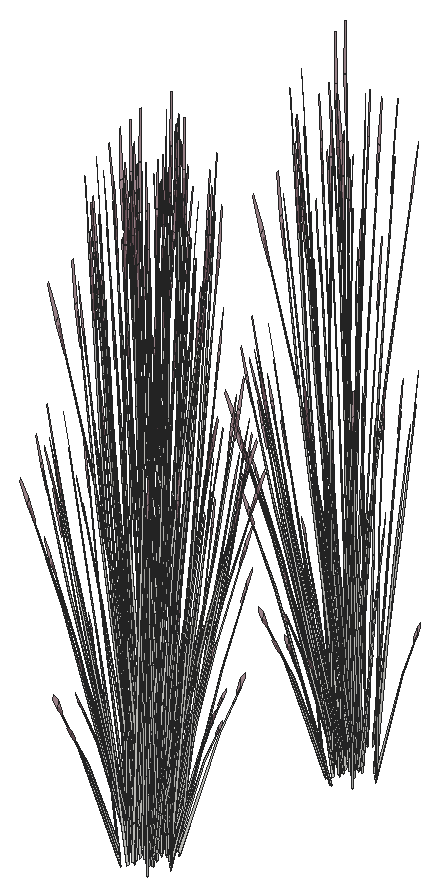
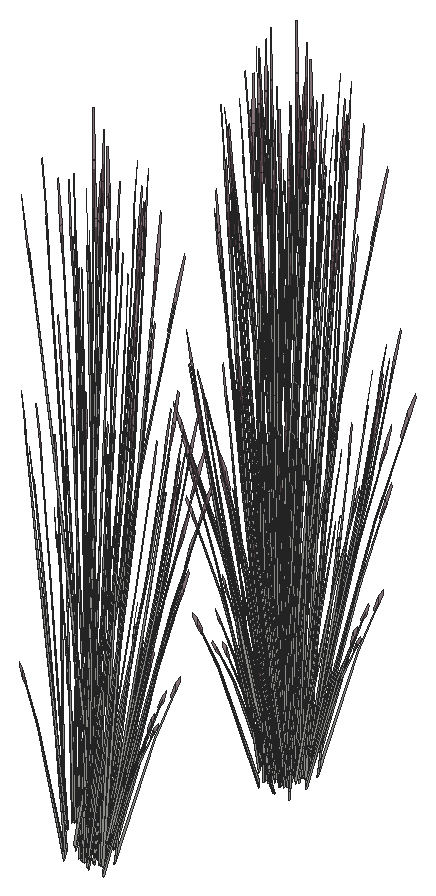
# SketchUp Ruby script. Lengths in inches.
U = 1.inch
M = Sketchup.active_model
def pt(a) = Geom::Point3d.new(a.map { |v| v * U })
def face(e, loops, mat)
  f = e.add_face(loops[0].map { |a| pt(a) })
  loops[1..].each { |l| e.add_face(l.map { |a| pt(a) }).erase! }
  f.material = f.back_material = mat if mat
  f
end
# faces: each face lists its corners as indices into pts; further lists are holes
def faces(e, pts, list, mat = nil) = list.each { |f| face(e, (f[0].is_a?(Array) ? f : [f]).map { |l| l.map { |i| pts[i] } }, mat) }
# xy, xz, yz: faces in a plane at the given z, y or x. An outline is a flat list of corners, or four numbers for a rectangle; further outlines are holes
def ring(l) = l.size == 4 ? [[l[0], l[1]], [l[2], l[1]], [l[2], l[3]], [l[0], l[3]]] : l.each_slice(2).to_a
def flat(e, list, mat, &to3) = list.each { |f| face(e, (f[0].is_a?(Array) ? f : [f]).map { |l| ring(l).map { |u, v| to3.(u, v) } }, mat) }
def xy(e, z, list, mat = nil) = flat(e, list, mat) { |x, y| [x, y, z] }
def xz(e, y, list, mat = nil) = flat(e, list, mat) { |x, z| [x, y, z] }
def yz(e, x, list, mat = nil) = flat(e, list, mat) { |y, z| [x, y, z] }
def lines(e, pts, list) = list.each { |a, b| e.add_line(pt(pts[a]), pt(pts[b])) }
# prism: a flat outline (further loops are holes) pulled along v
def prism(e, loops, v, mat = nil)
  f = face(e, loops, mat); d = Geom::Vector3d.new(v.map { |x| x * U })
  f.pushpull(f.normal.samedirection?(d) ? d.length : -d.length)
end
def box(e, o, s, mat = nil) = prism(e, [[o, [o[0] + s[0], o[1], o[2]], [o[0] + s[0], o[1] + s[1], o[2]], [o[0], o[1] + s[1], o[2]]]], [0, 0, s[2]], mat)
def at(x, y, z, deg = 0) = Geom::Transformation.translation(pt([x, y, z])) * Geom::Transformation.rotation(ORIGIN, Z_AXIS, deg.degrees)
def axes(o, x, y, z) = Geom::Transformation.new([*x, 0, *y, 0, *z, 0, *pt(o).to_a, 1])
def part(name) = M.definitions.add(name)
# library, detail: a bought-in or finely detailed component or shape, given as its bounding box
def library(name, o, s) = part(name).tap { |d| box(d.entities, o, s) }
def detail(e, o, s) = box(e.add_group.entities, o, s)
def put(e, d, t, mat = nil) = e.add_instance(d, t).tap { |i| i.material = mat if mat }
def group(e, t, mat = nil) = e.add_group.tap { |g| g.transformation = t; g.material = mat if mat }.entities
root = M.entities
M.materials.add("LightPink_Translucent").color = [144, 107, 117]
M.materials["LightPink_Translucent"].alpha = 0.75
c1 = part("blade")
p = [[2.15,0.21,22],[0,0.17,0],[0.09,0.45,0],[2.18,0.31,22],[2.29,0.31,22],[0.38,0.45,0],
  [2.48,0.24,33],[2.49,0.24,33],[2.48,0.22,33]]
faces(c1.entities,p,[[0,1,2,3],[4,5,2,3],[6,3,4,7],[8,0,3,6]])
c2 = part("seeds")
p = [[0.3,-0.1,1.38],[-0.01,-0.03,1.59],[-0.01,-0.03,0.03],[0.14,-0.07,-0.07],[0.29,-0.03,3],[0.15,0.01,3.11]]
faces(c2.entities,p,[[0,1,2,3],[1,0,4,5]],"LightPink_Translucent")
c3 = part("blade with seeds")
put(c3.entities,c1,at(0,0,0))
put(c3.entities,c2,axes([2.4,0.25,30.99],[1.5799,-0.05474,1.17369],[-0.12525,1.92788,0.29478],[-0.07173,-0.02425,1.56792]))
put(root,c3,axes([397.47,37.92,2.77],[0.18411,0.16231,1.1486],[-0.26813,0.09757,0.84392],[-0.05737,-0.12474,0.25299]))
put(root,c3,axes([397.91,38.78,4.98],[-0.30095,-0.22541,-0.71045],[0.21388,-0.395,0.08574],[-0.10904,-0.13459,1.00501]))
put(root,c3,axes([397.81,38.48,4.53],[-0.05451,-0.37564,-0.35414],[0.31161,-0.09919,0.4572],[-0.0837,-0.10765,0.87481]))
put(root,c3,axes([397.32,38.41,1.49],[-0.03419,0.06144,1.76342],[-0.3455,0.13246,-0.26939],[-0.08346,-0.12049,0.30037]))
put(root,c3,axes([397.89,40.1,2.1],[-0.14494,-0.47823,-0.69835],[0.41752,-0.17223,-0.18329],[-0.01602,-0.16194,1.54149]))
put(root,c3,axes([397.14,39.03,3.875],[0.1311,0.08035,1.71376],[-0.27131,0.33708,0.13857],[-0.16909,-0.15206,0.73262]))
put(root,c3,axes([399.83,38.64,1.49],[-0.05283,-0.03674,1.76342],[-0.13569,-0.41045,-0.26939],[0.09154,-0.11138,0.30037]))
put(root,c3,axes([397.77,38.79,4.68],[-0.34827,0.11086,-0.51099],[-0.06092,-0.41983,-0.3958],[-0.09354,-0.12031,0.97773]))
put(root,c3,axes([399.83,39.8,4.98],[0.18436,-0.36797,-0.71045],[0.32306,0.26151,0.08574],[0.11008,-0.13332,1.00501]))
put(root,c3,axes([397.83,38.72,2.375],[-0.22066,-0.46731,0],[0.36918,-0.26061,-0.51607],[0.08408,-0.05936,1.63711]))
put(root,c3,axes([399.82,39.625,4.68],[-0.09067,-0.42583,-0.51099],[0.34336,-0.07449,-0.3958],[0.0984,-0.11438,0.97773]))
put(root,c3,axes([398.32,38.16,2.13],[-0.2439,0.26754,-0.03893],[-0.22348,-0.29302,-0.17649],[-0.01573,-0.08303,0.58215]))
put(root,c3,axes([398.63,41.33,3.33],[0.305,0.18805,1.51261],[-0.29879,0.40513,0.59816],[-0.13384,-0.24012,1.26806]))
put(root,c3,axes([397.04,40.03,2.02],[0,-0.46636,-0.49651],[0.39487,0,0],[0,-0.10622,1.57504]))
put(root,c3,axes([398.13,38.65,2.02],[0.33032,-0.23318,-0.49651],[0.19744,0.41812,0],[0.07523,-0.05311,1.57504]))
put(root,c3,axes([400.09,39.46,2.59],[-0.12609,-0.01381,1.43002],[-0.12917,-0.37055,-0.30754],[0.1549,-0.10482,0.61141]))
put(root,c3,axes([398.53,39.61,2.06],[0.23773,-0.35053,-0.62353],[0.29532,0.31785,-0.16365],[0.09526,-0.08744,1.37633]))
put(root,c3,axes([400.24,38.78,2.77],[-0.11756,0.2374,1.1486],[-0.10105,-0.31895,0.84392],[0.09709,-0.07992,0.25299]))
put(root,c3,axes([400.07,39.67,4.53],[0.30722,-0.06665,-0.35414],[0.08112,0.381,0.4572],[0.08804,-0.10234,0.87481]))
put(root,c3,axes([398.11,40.22,2.21],[0.17124,-0.42022,-0.44739],[0.35581,0.20224,0.21531],[0,-0.09687,1.43643]))
put(root,c3,axes([397.09,39.15,4.53],[-0.20082,-0.29199,-0.35414],[0.2293,-0.2764,0.4572],[-0.1165,-0.04206,0.87481]))
put(root,c3,axes([398.27,40.01,2.67],[-0.04113,-0.53214,-0.29095],[0.42835,-0.03218,-0.50002],[0.07543,-0.07088,1.59708]))
put(root,c3,axes([397.21,40.04,2.03],[0.24637,-0.29097,-0.30978],[0.24637,0.29097,0.30978],[0,-0.09372,1.38974]))
put(root,c3,axes([397.11,38.65,2.13],[-0.10181,0.3808,-0.03893],[-0.31336,-0.11714,-0.17649],[-0.04758,-0.06228,0.58215]))
put(root,c3,axes([398.07,40.57,2.67],[-0.39748,-0.22252,-0.29095],[0.19139,-0.46966,-0.50002],[-0.01249,-0.11531,1.59708]))
put(root,c3,axes([396.9375,40.39,2.375],[-0.44133,0,0],[0,-0.52122,-0.51607],[0,-0.11871,1.63711]))
put(root,c3,axes([397.01,39.46,2.59],[0.06891,0.12984,1.43002],[-0.15879,0.35293,-0.30754],[-0.16304,-0.08436,0.61141]))
put(root,c3,axes([398.21,38.84,2.03],[0.32928,0.11539,-0.30978],[-0.08291,0.40636,0.30978],[0.06638,-0.04686,1.38974]))
put(root,c3,axes([397.3,39.34,4.98],[-0.35281,-0.01123,-0.71045],[0.0237,-0.47284,0.08574],[-0.14947,-0.0499,1.00501]))
put(root,c3,axes([397.28,40.25,2.33],[-0.32829,0.39208,0.30756],[-0.32849,-0.38796,-0.36492],[-0.01146,-0.11134,1.64885]))
put(root,c3,axes([398.32,40.43,2.43],[0.39767,0.22603,0.24065],[-0.19139,0.46966,0.50002],[0,-0.10827,1.60543]))
put(root,c3,axes([398.17,41.07,2.4375],[0.09355,-0.55261,-0.23429],[0.44354,0.09633,0.51271],[-0.0775,-0.07631,1.5644]))
put(root,c3,axes([397.18,39.4375,4.68],[-0.25628,0.30892,-0.51099],[-0.22444,-0.32634,-0.3958],[-0.13021,-0.047,0.97773]))
put(root,c3,axes([396.6,39.85,2.77],[0.22533,-0.03337,1.1486],[-0.14293,0.29403,0.84392],[-0.11135,-0.04411,0.25299]))
put(root,c3,axes([398.2,40.12,2.72],[-0.38326,0.02879,0.44739],[-0.03466,-0.47788,-0.21531],[0.06861,-0.04843,1.43643]))
put(root,c3,axes([397.21,40.47,2.48],[0,0.46636,0.49651],[-0.39487,0,0],[0,-0.10622,1.57504]))
put(root,c3,axes([399.98,40.57,4.68],[0.09562,-0.42421,-0.51099],[0.32782,0.1454,-0.3958],[0.13199,-0.0389,0.97773]))
put(root,c3,axes([399.46,38.84,2.375],[0.22066,-0.46731,0],[0.36918,0.26061,-0.51607],[0.08408,0.05936,1.63711]))
put(root,c3,axes([396.86,39.77,3.875],[0.14639,-0.01056,1.71376],[-0.09712,0.45778,0.13857],[-0.20862,-0.02831,0.73262]))
put(root,c3,axes([398.14,40.84,2.21],[-0.21202,-0.39143,-0.44739],[0.32115,-0.27564,0.21531],[-0.06861,-0.04843,1.43643]))
put(root,c3,axes([398.18,40.29,2.36],[0.15345,0.52148,0.45755],[-0.43845,0.18134,0.17955],[0.00536,-0.09582,1.58856]))
put(root,c3,axes([400.33,40.6875,1.98],[-0.22732,0.05597,1.41583],[-0.03618,-0.44548,0.08104],[0.15921,-0.06743,0.80566]))
put(root,c3,axes([400.74,40.29,2.26],[-0.21881,-0.29821,-0.06488],[0.23965,-0.27324,-0.29416],[0.0679,-0.01924,0.97024]))
put(root,c3,axes([398.1,40.7,2.72],[-0.17124,0.42022,0.44739],[-0.35581,-0.20224,-0.21531],[0,-0.09687,1.43643]))
put(root,c3,axes([398.73,40.33,2.21],[0,-0.53961,0],[0.44133,0,0],[0,0,1.79456]))
put(root,c3,axes([399.27,39.09,2.48],[-0.33032,-0.23318,0.49651],[0.19744,-0.41812,0],[0.07523,0.05311,1.57504]))
put(root,c3,axes([399.92,40.72,4.98],[0.31014,-0.20596,-0.71045],[0.17284,0.42397,0.08574],[0.14985,-0.04816,1.00501]))
put(root,c3,axes([397.95,40.99,2.06],[-0.36714,-0.07646,-0.62353],[0.07747,-0.47163,-0.16365],[-0.10956,-0.05715,1.37633]))
put(root,c3,axes([398.52,39.99,2.36],[-0.29264,0.42323,0.45755],[-0.34767,-0.3736,0.17955],[0.07055,-0.04224,1.58856]))
put(root,c3,axes([398.84,40.75,2.3],[-0.32829,-0.4014,-0.06131],[0.32849,-0.40164,0],[-0.01146,-0.01402,1.75571]))
put(root,c3,axes([398.02,39.3,2.47],[-0.10196,0.46348,0.17642],[-0.3731,-0.13116,0.35086],[0.06445,-0.00226,1.60407]))
put(root,c3,axes([397.86,39.67,1.59],[-0.3474,0.18671,1.28929],[-0.11057,-0.53572,0.50096],[0.21332,0.00891,1.46642]))
put(root,c3,axes([398.8,39.8125,2.62],[0.06809,-0.4162,0.1448],[0.33266,0.07225,-0.41347],[0.06054,0.04274,1.26744]))
put(root,c3,axes([398.22,40.8,2.36],[0.44609,0.09826,0.45755],[-0.09078,0.55493,0.17955],[-0.06519,-0.05359,1.58856]))
put(root,c3,axes([400.58,40.4,1.49],[-0.01845,-0.0708,1.76342],[0.12793,-0.41416,-0.26939],[0.12905,-0.00596,0.30037]))
put(root,c3,axes([396.77,40.33,1.49],[0.00895,0.0735,1.76342],[-0.18044,0.38382,-0.26939],[-0.12817,-0.01935,0.30037]))
put(root,c3,axes([398.65,39.92,2.72],[-0.21202,-0.39143,0.44739],[0.32115,-0.27564,-0.21531],[0.06861,0.04843,1.43643]))
put(root,c3,axes([397.56,41.71,2.03],[-0.08291,-0.40636,-0.30978],[0.32928,-0.11539,0.30978],[-0.06638,-0.04686,1.38974]))
put(root,c3,axes([397.98,41.6875,2.47],[0.37926,-0.12378,0.17642],[0.09365,0.46065,0.35086],[-0.03382,-0.06712,1.60407]))
put(root,c3,axes([398.76,39.95,2.67],[0.35635,-0.30962,-0.29095],[0.23697,0.43749,-0.50002],[0.08792,0.04443,1.59708]))
put(root,c3,axes([400.18,40.76,4.53],[0.29332,0.1301,-0.35414],[-0.08555,0.37955,0.4572],[0.11809,-0.0348,0.87481]))
put(root,c3,axes([397.47,41.88,2.02],[-0.33032,-0.23318,-0.49651],[0.19744,-0.41812,0],[-0.07523,-0.05311,1.57504]))
put(root,c3,axes([399.66,39.125,2.02],[0.33032,0.23318,-0.49651],[-0.19744,0.41812,0],[0.07523,0.05311,1.57504]))
put(root,c3,axes([396.73,40.16,4.53],[-0.29332,-0.1301,-0.35414],[0.08555,-0.37955,0.4572],[-0.11809,0.0348,0.87481]))
put(root,c3,axes([399.03,40.45,2.21],[0.39487,0,0],[0,0.48281,0],[0,0,1.78407]))
put(root,c3,axes([398.36,41.0625,2.67],[-0.35635,0.30962,-0.29095],[-0.23697,-0.43749,-0.50002],[-0.08792,-0.04443,1.59708]))
put(root,c3,axes([399.15,39.32,2.47],[-0.37926,0.12378,0.17642],[-0.09365,-0.46065,0.35086],[0.03382,0.06712,1.60407]))
put(root,c3,axes([399.38,40.29,3.875],[-0.14639,0.01056,1.71376],[0.09712,-0.45778,0.13857],[0.20862,0.02831,0.73262]))
put(root,c3,axes([399.57,39.3,2.03],[0.08291,0.40636,-0.30978],[-0.32928,0.11539,0.30978],[0.06638,0.04686,1.38974]))
put(root,c3,axes([398.91,40.21,2.38],[-0.44609,-0.09826,0.49198],[0.09078,-0.55493,0.19306],[0.06519,0.05359,1.70813]))
put(root,c3,axes([398.55,41.58,2.2],[-0.11516,-0.40207,0],[0.32884,-0.1408,0],[0,0,1.54371]))
put(root,c3,axes([398.33,41.2,2.62],[-0.06809,0.4162,0.1448],[-0.33266,-0.07225,-0.41347],[-0.06054,-0.04274,1.26744]))
put(root,c3,axes([398.98,41.52,2.18],[0.37054,-0.15823,-0.19198],[0.1302,0.45581,0.00008],[0.0409,-0.01749,1.73897]))
put(root,c3,axes([399.11,41.71,2.47],[0.10196,-0.46348,0.17642],[0.3731,0.13116,0.35086],[-0.06445,0.00226,1.60407]))
put(root,c3,axes([399.02,40.66,2.21],[0.24637,0.30123,0],[-0.24637,0.30123,0],[0,0,1.69266]))
put(root,c3,axes([397.625,40.1,3.34],[0.10032,-0.06746,1.77064],[0.0346,0.47103,0.13857],[-0.2173,0.0625,0.63284]))
put(root,c3,axes([399.69,40.53,2.47],[-0.2773,-0.3397,0.17642],[0.27945,-0.32949,0.35086],[-0.03063,0.06937,1.60407]))
put(root,c3,axes([399.18,40.02,2.06],[0.36714,0.07646,-0.62353],[-0.07747,0.47163,-0.16365],[0.10956,0.05715,1.37633]))
put(root,c3,axes([400.8,40.84,2.77],[-0.21807,0.07699,1.1486],[0.10265,-0.31819,0.84392],[0.11568,0.02177,0.25299]))
put(root,c3,axes([398.47,41.76,2.2],[-0.35581,-0.20937,0],[0.17124,-0.43505,0],[0,0,1.62707]))
put(root,c3,axes([398.76,41.2,2.46],[-0.34464,-0.37536,-0.25192],[0.29,-0.42149,0.5513],[-0.0928,0.04391,1.68216]))
put(root,c3,axes([397.86,41.92,2.48],[0.33032,0.23318,0.49651],[-0.19744,0.41812,0],[-0.07523,-0.05311,1.57504]))
put(root,c3,axes([399.02,40.31,2.72],[0.17124,-0.42022,0.44739],[0.35581,0.20224,-0.21531],[0,0.09687,1.43643]))
put(root,c3,axes([398.96,40.55,2.29],[0,0.53934,-0.05637],[-0.44133,0,0],[0,0.01695,1.79368]))
put(root,c3,axes([396.93,40.35,4.68],[-0.09562,0.42421,-0.51099],[-0.32782,-0.1454,-0.3958],[-0.13199,0.0389,0.97773]))
put(root,c3,axes([398.99,40.17,2.21],[0.21202,0.39143,-0.44739],[-0.32115,0.27564,0.21531],[0.06861,0.04843,1.43643]))
put(root,c3,axes([400.42,41.82,3.93],[-0.06755,-0.39203,-0.03492],[0.31928,-0.09013,-0.15832],[0.06667,0.02485,0.52218]))
put(root,c3,axes([397.67,42.17,2.375],[-0.22066,0.46731,0],[-0.36918,-0.26061,-0.51607],[-0.08408,-0.05936,1.63711]))
put(root,c3,axes([399.92,40.54,2.48],[0,-0.46636,0.49651],[0.39487,0,0],[0,0.10622,1.57504]))
put(root,c3,axes([398.93,40.89,2.72],[0.38326,-0.02879,0.44739],[0.03466,0.47788,-0.21531],[-0.06861,0.04843,1.43643]))
put(root,c3,axes([399.17,40.4,2.62],[0.32884,-0.136,0.1448],[0.11516,0.38837,-0.41347],[0,0.08547,1.26744]))
put(root,c3,axes([398.59,41.125,2.21],[-0.38326,0.02879,-0.44739],[-0.03466,-0.47788,0.21531],[-0.06861,0.04843,1.43643]))
put(root,c3,axes([400.39,41.35,2.59],[-0.085,-0.1147,1.43002],[0.1106,-0.37943,-0.30754],[0.17198,0.0514,0.61141]))
put(root,c3,axes([398.87,41.77,2.2],[0.35581,0.20937,0],[-0.17124,0.43505,0],[0,0,1.74954]))
put(root,c3,axes([399.01,42.23,2.19],[-0.21791,-0.46895,-0.05142],[0.36918,-0.26061,0.51607],[-0.09097,0.04465,1.6363]))
put(root,c3,axes([398.9375,41.1,2.62],[0.26075,0.2802,0.1448],[-0.2175,0.31612,-0.41347],[-0.06054,0.04274,1.26744]))
put(root,c3,axes([396.92,40.57,3.875],[0.12246,-0.09864,1.71376],[0.1031,0.45582,0.13857],[-0.19225,0.10302,0.73262]))
put(root,c3,axes([399.61,41.58,4.98],[0.35281,0.01123,-0.71045],[-0.0237,0.47284,0.08574],[0.14947,0.0499,1.00501]))
put(root,c3,axes([399.21,41.96,2.48],[0.33032,-0.23318,0.49651],[0.19744,0.41812,0],[-0.07523,0.05311,1.57504]))
put(root,c3,axes([398.74,41.59,2.29],[0.15345,0.53576,-0.06012],[-0.43845,0.18773,0],[0.00536,0.01871,1.72173]))
put(root,c3,axes([398.91,42.17,2.03],[-0.32928,-0.11539,-0.30978],[0.08291,-0.40636,0.30978],[-0.06638,0.04686,1.38974]))
put(root,c3,axes([396.54,41.35,2.59],[0.12266,0.03828,1.43002],[0.07906,0.39104,-0.30754],[-0.16661,0.0732,0.61141]))
put(root,c3,axes([400.1875,40.62,2.375],[0.44133,0,0],[0,0.52122,-0.51607],[0,0.11871,1.63711]))
put(root,c3,axes([400.01,40.89,2.2],[-0.44111,-0.00373,-0.04976],[0,-0.52122,0.49943],[-0.01386,0.11865,1.58352]))
put(root,c3,axes([399.06,40.4375,2.67],[0.39748,0.22252,-0.29095],[-0.19139,0.46966,-0.50002],[0.01249,0.11531,1.59708]))
put(root,c3,axes([396.28,42.17,2.77],[0.14709,-0.21136,1.1486],[0.05804,0.3346,0.84392],[-0.1063,0.05991,0.25299]))
put(root,c3,axes([399.82,41.78,4.53],[0.20082,0.29199,-0.35414],[-0.2293,0.2764,0.4572],[0.1165,0.04206,0.87481]))
put(root,c3,axes([399.92,40.97,2.03],[-0.24637,0.29097,-0.30978],[-0.24637,-0.29097,0.30978],[0,0.09372,1.38974]))
put(root,c3,axes([398.86,40.99,2.67],[0.04113,0.53214,-0.29095],[-0.42835,0.03218,-0.50002],[-0.07543,0.07088,1.59708]))
put(root,c3,axes([399.01,40.79,2.21],[-0.17124,0.42022,-0.44739],[-0.35581,-0.20224,0.21531],[0,0.09687,1.43643]))
put(root,c3,axes([396.84,41.25,4.53],[-0.30722,0.06665,-0.35414],[-0.08112,-0.381,0.4572],[-0.08804,0.10234,0.87481]))
put(root,c3,axes([398.6,41.4,2.06],[-0.23773,0.35053,-0.62353],[-0.29532,-0.31785,-0.16365],[-0.09526,0.08744,1.37633]))
put(root,c3,axes([399.02,41.99,2.33],[0.44186,0.15158,0.30756],[-0.11054,0.54181,-0.36492],[-0.07313,0.06781,1.64885]))
put(root,c3,axes([398.99,42.36,2.02],[-0.33032,0.23318,-0.49651],[-0.19744,-0.41812,0],[-0.07523,0.05311,1.57504]))
put(root,c3,axes([400.09,40.98,2.02],[0,0.46636,-0.49651],[-0.39487,0,0],[0,0.10622,1.57504]))
put(root,c3,axes([399.1,41.03,3.875],[-0.1311,-0.08035,1.71376],[0.27131,-0.33708,0.13857],[0.16909,0.15206,0.73262]))
put(root,c3,axes([399.59,41.94,2.77],[-0.19872,-0.13409,1.1486],[0.2566,-0.13625,0.84392],[0.06921,0.11541,0.25299]))
put(root,c3,axes([397.37,40.88,3.875],[0.08815,-0.14329,1.71376],[0.22258,0.38678,0.13857],[-0.15267,0.17614,0.73262]))
put(root,c3,axes([397.09,41.3,4.68],[0.09067,0.42583,-0.51099],[-0.34336,0.07449,-0.3958],[-0.0984,0.11438,0.97773]))
put(root,c3,axes([399.29,42.28,2.375],[0.22066,0.46731,0],[-0.36918,0.26061,-0.51607],[-0.08408,0.05936,1.63711]))
put(root,c3,axes([399.64,42.44,1.49],[0.02571,-0.06733,1.76342],[0.32373,-0.19829,-0.26939],[0.09815,0.10263,0.30037]))
put(root,c3,axes([399.1,40.43,2.84],[-0.00964,-0.43909,1.41272],[0.43635,0.11382,0.59816],[-0.1032,0.24027,1.3335]))
put(root,c3,axes([399.22,40.91,2.09],[0.12941,0.42699,-0.69212],[-0.37279,0.15378,-0.18165],[0.0143,0.14459,1.52773]))
put(root,c3,axes([396.67,42.38,1.49],[0.04734,0.04659,1.76342],[0.08027,0.4317,-0.26939],[-0.10492,0.09206,0.30037]))
put(root,c3,axes([399.14,42.13,4.68],[0.34827,-0.11086,-0.51099],[0.06092,0.41983,-0.3958],[0.09354,0.12031,0.97773]))
put(root,c3,axes([399.62,42.55,2.67],[-0.22633,-0.01463,1.0506],[0.14947,-0.31064,0.58006],[0.08941,0.11036,0.8241]))
put(root,c3,axes([397.3,41.23,3.875],[0.06572,-0.16029,1.71376],[0.27569,0.33172,0.13857],[-0.12437,0.20675,0.73262]))
put(root,c3,axes([398.88,41.8,2.59],[0.00623,-0.15459,1.43002],[0.29764,-0.17268,-0.30754],[0.09188,0.18503,0.61141]))
put(root,c3,axes([397.38,42.14,4.53],[-0.23881,0.24554,-0.35414],[-0.22606,-0.28036,0.4572],[-0.0344,0.14245,0.87481]))
put(root,c3,axes([397.53,43.09,2.77],[-0.00913,-0.2773,1.1486],[0.22824,0.19778,0.84392],[-0.04489,0.13217,0.25299]))
put(root,c3,axes([398.13,42.43,1.49],[0.05712,-0.02538,1.76342],[0.34359,0.13968,-0.26939],[0.01005,0.15742,0.30037]))
put(root,c3,axes([397.62,42.02,5],[0.25266,0.31335,-0.5672],[-0.2669,0.27442,-0.43934],[-0.03844,0.15921,1.08528]))
put(root,c3,axes([397.34,42.49,2.82],[0.32063,-0.08258,0.06507],[0.07371,0.33271,-0.86304],[-0.02033,0.16842,0.7736]))
put(root,c3,axes([398.37,42.32,4.68],[0.34695,0.11691,-0.51099],[-0.11892,0.40083,-0.3958],[0.03181,0.16138,0.97773]))
put(root,c3,axes([398.5625,41.5,3.875],[-0.08068,-0.14973,1.71376],[0.3728,-0.12606,0.13857],[0.08426,0.23506,0.73262]))
put(root,c3,axes([398.21,42.57,4.53],[-0.1064,0.35863,-0.35414],[-0.31043,-0.1046,0.4572],[0.02846,0.14439,0.87481]))
put(root,c3,axes([397.54,41.875,5.34],[-0.00918,0.43138,-0.7886],[-0.38672,-0.02897,0.09517],[-0.04081,0.18275,1.11556]))
put(root,c3,axes([397.9,41.57,3.875],[-0.00864,-0.17899,1.71376],[0.37441,0.11874,0.13857],[-0.02316,0.25508,0.73262]))
put(root,c3,axes([398.24,42.25,4.98],[0.16845,0.3792,-0.71045],[-0.34676,0.21133,0.08574],[0.03939,0.18322,1.00501]))
put(root,c3,axes([397.26,42.84,2.59],[0.11138,-0.07357,1.43002],[0.27499,0.22183,-0.30754],[-0.08185,0.19194,0.61141]))
put(root,c3,axes([397.41,42.48,3.36],[0.00775,-0.24075,1.54345],[0.34877,0.12716,0.21329],[-0.03022,0.25658,0.72882]))
put(root,c3,axes([401.27,58.66,3.875],[0.08068,0.14973,1.71376],[-0.3728,0.12606,0.13857],[-0.08426,-0.23506,0.73262]))
put(root,c3,axes([402.72,58.44,2.59],[-0.10032,0.0944,1.43002],[-0.30046,-0.16522,-0.30754],[0.05569,-0.20547,0.61141]))
put(root,c3,axes([402.27,58.77,4.98],[-0.16845,-0.3792,-0.71045],[0.34676,-0.21133,0.08574],[-0.03939,-0.18322,1.00501]))
put(root,c3,axes([401.17,58.26,2.59],[-0.02137,0.15256,1.43002],[-0.31245,0.12771,-0.30754],[-0.07303,-0.19719,0.61141]))
put(root,c3,axes([401.98,57.93,1.49],[-0.0592,0.0168,1.76342],[-0.32738,-0.18913,-0.26939],[0.00549,-0.15776,0.30037]))
put(root,c3,axes([402.97,59.14,4.98],[0.00918,-0.43138,-0.71045],[0.38672,0.02897,0.08574],[0.04081,-0.18275,1.00501]))
put(root,c3,axes([402.3,58.45,4.53],[0.1064,-0.35863,-0.35414],[0.31043,0.1046,0.4572],[-0.02846,-0.14439,0.87481]))
put(root,c3,axes([402.53,58.92,3.875],[-0.06572,0.16029,1.71376],[-0.27569,-0.33172,0.13857],[0.12437,-0.20675,0.73262]))
put(root,c3,axes([402.14,58.69,4.68],[-0.34695,-0.11691,-0.51099],[0.11892,-0.40083,-0.3958],[-0.03181,-0.16138,0.97773]))
put(root,c3,axes([402.35,57.69,2.77],[0.04528,0.27194,1.1486],[-0.25117,-0.15062,0.84392],[0.02703,-0.13924,0.25299]))
put(root,c3,axes([402.89,59,4.68],[-0.25266,-0.31335,-0.51099],[0.2669,-0.27442,-0.3958],[0.03844,-0.15921,0.97773]))
put(root,c3,axes([403.13,58.88,4.53],[0.23881,-0.24554,-0.35414],[0.22606,0.28036,0.4572],[0.0344,-0.14245,0.87481]))
put(root,c3,axes([401.0625,58.02,2.77],[0.18411,0.16231,1.1486],[-0.26813,0.09757,0.84392],[-0.05737,-0.12474,0.25299]))
put(root,c3,axes([401.51,58.88,4.98],[-0.30095,-0.22541,-0.71045],[0.21388,-0.395,0.08574],[-0.10904,-0.13459,1.00501]))
put(root,c3,axes([401.4,58.58,4.53],[-0.05451,-0.37564,-0.35414],[0.31161,-0.09919,0.4572],[-0.0837,-0.10765,0.87481]))
put(root,c3,axes([400.92,58.51,1.49],[-0.03419,0.06144,1.76342],[-0.3455,0.13246,-0.26939],[-0.08346,-0.12049,0.30037]))
put(root,c3,axes([401.49,60.2,2.1],[-0.14494,-0.47823,-0.69835],[0.41752,-0.17223,-0.18329],[-0.01602,-0.16194,1.54149]))
put(root,c3,axes([400.73,59.125,3.875],[0.1311,0.08035,1.71376],[-0.27131,0.33708,0.13857],[-0.16909,-0.15206,0.73262]))
put(root,c3,axes([403.43,58.73,1.49],[-0.05283,-0.03674,1.76342],[-0.13569,-0.41045,-0.26939],[0.09154,-0.11138,0.30037]))
put(root,c3,axes([401.37,58.89,4.68],[-0.34827,0.11086,-0.51099],[-0.06092,-0.41983,-0.3958],[-0.09354,-0.12031,0.97773]))
put(root,c3,axes([403.42,59.89,4.98],[0.18436,-0.36797,-0.71045],[0.32306,0.26151,0.08574],[0.11008,-0.13332,1.00501]))
put(root,c3,axes([401.43,58.82,2.375],[-0.22066,-0.46731,0],[0.36918,-0.26061,-0.51607],[0.08408,-0.05936,1.63711]))
put(root,c3,axes([403.41,59.72,4.68],[-0.09067,-0.42583,-0.51099],[0.34336,-0.07449,-0.3958],[0.0984,-0.11438,0.97773]))
put(root,c3,axes([401.92,58.26,2.13],[-0.2439,0.26754,-0.03893],[-0.22348,-0.29302,-0.17649],[-0.01573,-0.08303,0.58215]))
put(root,c3,axes([402.23,61.43,3.33],[0.305,0.18805,1.51261],[-0.29879,0.40513,0.59816],[-0.13384,-0.24012,1.26806]))
put(root,c3,axes([400.63,60.13,2.02],[0,-0.46636,-0.49651],[0.39487,0,0],[0,-0.10622,1.57504]))
put(root,c3,axes([401.73,58.75,2.02],[0.33032,-0.23318,-0.49651],[0.19744,0.41812,0],[0.07523,-0.05311,1.57504]))
put(root,c3,axes([403.69,59.55,2.59],[-0.12609,-0.01381,1.43002],[-0.12917,-0.37055,-0.30754],[0.1549,-0.10482,0.61141]))
put(root,c3,axes([402.12,59.7,2.06],[0.23773,-0.35053,-0.62353],[0.29532,0.31785,-0.16365],[0.09526,-0.08744,1.37633]))
put(root,c3,axes([403.84,58.87,2.77],[-0.11756,0.2374,1.1486],[-0.10105,-0.31895,0.84392],[0.09709,-0.07992,0.25299]))
put(root,c3,axes([403.67,59.76,4.53],[0.30722,-0.06665,-0.35414],[0.08112,0.381,0.4572],[0.08804,-0.10234,0.87481]))
put(root,c3,axes([401.71,60.32,2.21],[0.17124,-0.42022,-0.44739],[0.35581,0.20224,0.21531],[0,-0.09687,1.43643]))
put(root,c3,axes([400.68,59.24,4.53],[-0.20082,-0.29199,-0.35414],[0.2293,-0.2764,0.4572],[-0.1165,-0.04206,0.87481]))
put(root,c3,axes([401.86,60.11,2.67],[-0.04113,-0.53214,-0.29095],[0.42835,-0.03218,-0.50002],[0.07543,-0.07088,1.59708]))
put(root,c3,axes([400.8,60.14,2.03],[0.24637,-0.29097,-0.30978],[0.24637,0.29097,0.30978],[0,-0.09372,1.38974]))
put(root,c3,axes([400.7,58.74,2.13],[-0.10181,0.3808,-0.03893],[-0.31336,-0.11714,-0.17649],[-0.04758,-0.06228,0.58215]))
put(root,c3,axes([401.67,60.67,2.67],[-0.39748,-0.22252,-0.29095],[0.19139,-0.46966,-0.50002],[-0.01249,-0.11531,1.59708]))
put(root,c3,axes([400.53,60.48,2.375],[-0.44133,0,0],[0,-0.52122,-0.51607],[0,-0.11871,1.63711]))
put(root,c3,axes([400.61,59.55,2.59],[0.06891,0.12984,1.43002],[-0.15879,0.35293,-0.30754],[-0.16304,-0.08436,0.61141]))
put(root,c3,axes([401.81,58.93,2.03],[0.32928,0.11539,-0.30978],[-0.08291,0.40636,0.30978],[0.06638,-0.04686,1.38974]))
put(root,c3,axes([400.89,59.4375,4.98],[-0.35281,-0.01123,-0.71045],[0.0237,-0.47284,0.08574],[-0.14947,-0.0499,1.00501]))
put(root,c3,axes([400.875,60.34,2.33],[-0.32829,0.39208,0.30756],[-0.32849,-0.38796,-0.36492],[-0.01146,-0.11134,1.64885]))
put(root,c3,axes([401.92,60.53,2.43],[0.39767,0.22603,0.24065],[-0.19139,0.46966,0.50002],[0,-0.10827,1.60543]))
put(root,c3,axes([401.77,61.16,2.4375],[0.09355,-0.55261,-0.23429],[0.44354,0.09633,0.51271],[-0.0775,-0.07631,1.5644]))
put(root,c3,axes([400.78,59.53,4.68],[-0.25628,0.30892,-0.51099],[-0.22444,-0.32634,-0.3958],[-0.13021,-0.047,0.97773]))
put(root,c3,axes([400.2,59.94,2.77],[0.22533,-0.03337,1.1486],[-0.14293,0.29403,0.84392],[-0.11135,-0.04411,0.25299]))
put(root,c3,axes([401.79,60.21,2.72],[-0.38326,0.02879,0.44739],[-0.03466,-0.47788,-0.21531],[0.06861,-0.04843,1.43643]))
put(root,c3,axes([400.8,60.5625,2.48],[0,0.46636,0.49651],[-0.39487,0,0],[0,-0.10622,1.57504]))
put(root,c3,axes([403.57,60.67,4.68],[0.09562,-0.42421,-0.51099],[0.32782,0.1454,-0.3958],[0.13199,-0.0389,0.97773]))
put(root,c3,axes([403.06,58.9375,2.375],[0.22066,-0.46731,0],[0.36918,0.26061,-0.51607],[0.08408,0.05936,1.63711]))
put(root,c3,axes([400.46,59.86,3.875],[0.14639,-0.01056,1.71376],[-0.09712,0.45778,0.13857],[-0.20862,-0.02831,0.73262]))
put(root,c3,axes([401.73,60.9375,2.21],[-0.21202,-0.39143,-0.44739],[0.32115,-0.27564,0.21531],[-0.06861,-0.04843,1.43643]))
put(root,c3,axes([401.78,60.39,2.36],[0.15345,0.52148,0.45755],[-0.43845,0.18134,0.17955],[0.00536,-0.09582,1.58856]))
put(root,c3,axes([403.92,60.79,1.98],[-0.22732,0.05597,1.41583],[-0.03618,-0.44548,0.08104],[0.15921,-0.06743,0.80566]))
put(root,c3,axes([404.34,60.39,2.26],[-0.21881,-0.29821,-0.06488],[0.23965,-0.27324,-0.29416],[0.0679,-0.01924,0.97024]))
put(root,c3,axes([401.7,60.8,2.72],[-0.17124,0.42022,0.44739],[-0.35581,-0.20224,-0.21531],[0,-0.09687,1.43643]))
put(root,c3,axes([402.33,60.43,2.21],[0,-0.53961,0],[0.44133,0,0],[0,0,1.79456]))
put(root,c3,axes([402.87,59.18,2.48],[-0.33032,-0.23318,0.49651],[0.19744,-0.41812,0],[0.07523,0.05311,1.57504]))
put(root,c3,axes([403.51,60.82,4.98],[0.31014,-0.20596,-0.71045],[0.17284,0.42397,0.08574],[0.14985,-0.04816,1.00501]))
put(root,c3,axes([401.54,61.09,2.06],[-0.36714,-0.07646,-0.62353],[0.07747,-0.47163,-0.16365],[-0.10956,-0.05715,1.37633]))
put(root,c3,axes([402.12,60.09,2.36],[-0.29264,0.42323,0.45755],[-0.34767,-0.3736,0.17955],[0.07055,-0.04224,1.58856]))
put(root,c3,axes([402.44,60.85,2.3],[-0.32829,-0.4014,-0.06131],[0.32849,-0.40164,0],[-0.01146,-0.01402,1.75571]))
put(root,c3,axes([401.61,59.39,2.47],[-0.10196,0.46348,0.17642],[-0.3731,-0.13116,0.35086],[0.06445,-0.00226,1.60407]))
put(root,c3,axes([401.46,59.77,1.59],[-0.3474,0.18671,1.28929],[-0.11057,-0.53572,0.50096],[0.21332,0.00891,1.46642]))
put(root,c3,axes([402.39,59.91,2.62],[0.06809,-0.4162,0.1448],[0.33266,0.07225,-0.41347],[0.06054,0.04274,1.26744]))
put(root,c3,axes([401.82,60.9,2.36],[0.44609,0.09826,0.45755],[-0.09078,0.55493,0.17955],[-0.06519,-0.05359,1.58856]))
put(root,c3,axes([404.17,60.49,1.49],[-0.01845,-0.0708,1.76342],[0.12793,-0.41416,-0.26939],[0.12905,-0.00596,0.30037]))
put(root,c3,axes([400.36,60.42,1.49],[0.00895,0.0735,1.76342],[-0.18044,0.38382,-0.26939],[-0.12817,-0.01935,0.30037]))
